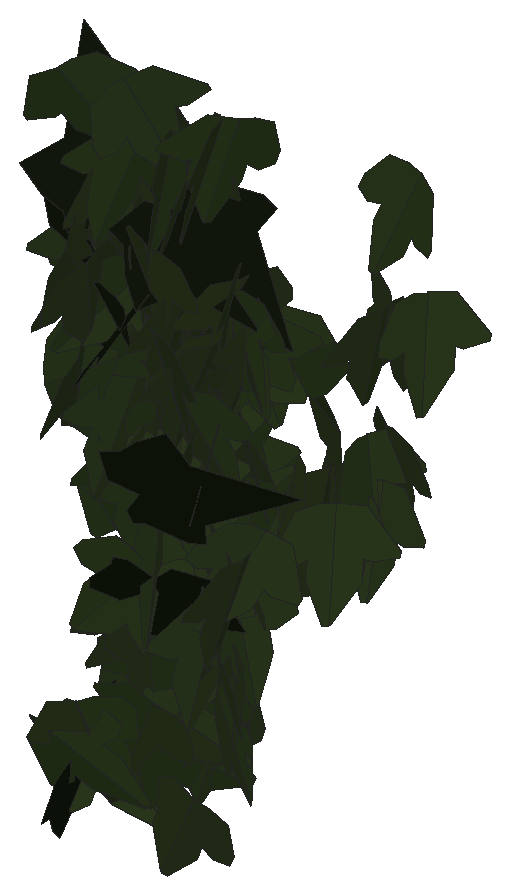
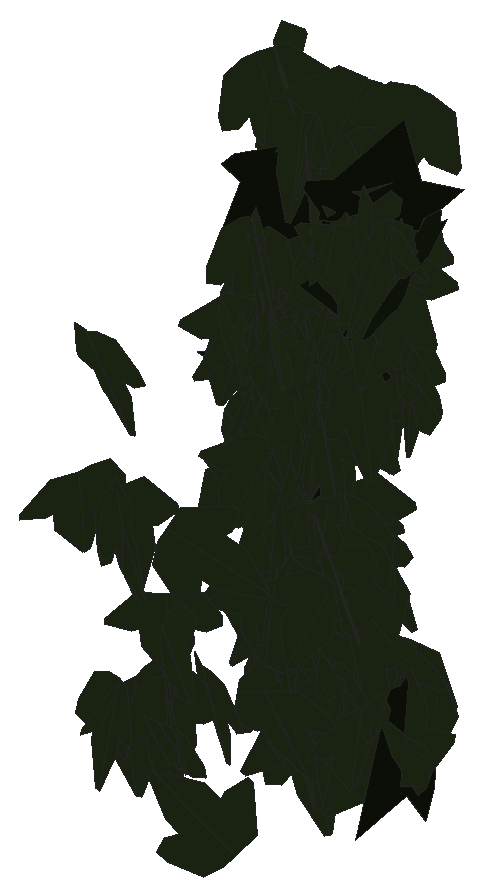
# SketchUp Ruby script. Lengths in inches.
U = 1.inch
M = Sketchup.active_model
def pt(a) = Geom::Point3d.new(a.map { |v| v * U })
def face(e, loops, mat)
  f = e.add_face(loops[0].map { |a| pt(a) })
  loops[1..].each { |l| e.add_face(l.map { |a| pt(a) }).erase! }
  f.material = f.back_material = mat if mat
  f
end
# faces: each face lists its corners as indices into pts; further lists are holes
def faces(e, pts, list, mat = nil) = list.each { |f| face(e, (f[0].is_a?(Array) ? f : [f]).map { |l| l.map { |i| pts[i] } }, mat) }
# xy, xz, yz: faces in a plane at the given z, y or x. An outline is a flat list of corners, or four numbers for a rectangle; further outlines are holes
def ring(l) = l.size == 4 ? [[l[0], l[1]], [l[2], l[1]], [l[2], l[3]], [l[0], l[3]]] : l.each_slice(2).to_a
def flat(e, list, mat, &to3) = list.each { |f| face(e, (f[0].is_a?(Array) ? f : [f]).map { |l| ring(l).map { |u, v| to3.(u, v) } }, mat) }
def xy(e, z, list, mat = nil) = flat(e, list, mat) { |x, y| [x, y, z] }
def xz(e, y, list, mat = nil) = flat(e, list, mat) { |x, z| [x, y, z] }
def yz(e, x, list, mat = nil) = flat(e, list, mat) { |y, z| [x, y, z] }
def lines(e, pts, list) = list.each { |a, b| e.add_line(pt(pts[a]), pt(pts[b])) }
# prism: a flat outline (further loops are holes) pulled along v
def prism(e, loops, v, mat = nil)
  f = face(e, loops, mat); d = Geom::Vector3d.new(v.map { |x| x * U })
  f.pushpull(f.normal.samedirection?(d) ? d.length : -d.length)
end
def box(e, o, s, mat = nil) = prism(e, [[o, [o[0] + s[0], o[1], o[2]], [o[0] + s[0], o[1] + s[1], o[2]], [o[0], o[1] + s[1], o[2]]]], [0, 0, s[2]], mat)
def at(x, y, z, deg = 0) = Geom::Transformation.translation(pt([x, y, z])) * Geom::Transformation.rotation(ORIGIN, Z_AXIS, deg.degrees)
def axes(o, x, y, z) = Geom::Transformation.new([*x, 0, *y, 0, *z, 0, *pt(o).to_a, 1])
def part(name) = M.definitions.add(name)
# library, detail: a bought-in or finely detailed component or shape, given as its bounding box
def library(name, o, s) = part(name).tap { |d| box(d.entities, o, s) }
def detail(e, o, s) = box(e.add_group.entities, o, s)
def put(e, d, t, mat = nil) = e.add_instance(d, t).tap { |i| i.material = mat if mat }
def group(e, t, mat = nil) = e.add_group.tap { |g| g.transformation = t; g.material = mat if mat }.entities
root = M.entities
M.materials.add("efeu1").color = [18, 25, 13]
M.materials.add("efeu2").color = [43, 57, 29]
c1 = part("ivyleaf_10")
p = [[0,0.5,-0.03],[-0.0625,2.02,-0.43],[-0.19,2.01,-0.46],[-0.54,1.05,-0.29],[-0.52,0.625,-0.18],[-0.83,0.76,-0.28],
  [-1.16,0.64,-0.33],[-1.15,0.33,-0.24],[-0.77,-0.39,0.02],[-0.3,-0.51,0.16],[0.04,-0.48,0.23],[-0.02,2.01,-0.4375],
  [-0.06,2.01,-0.43],[0.04,-0.49,0.23],[0.67,-0.49,0.14],[1.38,0.36,-0.2],[1.375,0.51,-0.24],[0.81,0.65,-0.19],
  [0.62,0.59,-0.15],[0.6,1.09,-0.28],[0.5,1.23,-0.31]]
faces(c1.entities,p,[[0,1,2,3,4,5,6,7,8,9,10],[11,12,0,13,14,15,16,17,18,19,20]],"efeu2")
c2 = part("ivyleaf_9")
p = [[1.54,2.16,1.25],[1.36,2.04,1.19],[-0.21,0.99,0.68],[-0.71,1.11,0.82],[-0.85,0.86,0.67],[-0.8,0.17,0.21],
  [-0.9,-0.01,0.1],[-0.67,-0.16,-0.02],[-0.08,-0.08,-0.05],[-0.03,-0.6,-0.4],[0.65,-0.88,-0.66],[0.83,-0.6,-0.49],
  [1.29,-0.42,-0.43],[1.8125,-0.07,-0.26],[1.21,0.44,0.15]]
faces(c2.entities,p,[[0,1,2,3,4,5,6,7,8,9,10,11,12,13,14]],"efeu1")
put(root,c1,axes([524.13,137.27,180.83],[-0.47127,-0.50798,0.10975],[-0.01474,-0.13503,-0.68828],[0.51949,-0.46466,0.08003]))
put(root,c1,axes([523.68,138.11,176.34],[-0.41982,-0.07668,-0.5031],[0.50786,-0.0214,-0.42054],[0.03256,-0.6549,0.07265]))
put(root,c2,axes([524.28,136.52,173],[-0.12797,0.15475,-0.77354],[-0.54598,0.54826,0.2],[0.5694,0.56049,0.01793]))
put(root,c1,axes([524.01,137.43,181.48],[0.01965,-0.59176,-0.37503],[0.17898,0.36697,-0.56966],[0.67734,-0.0798,0.16141]))
put(root,c1,axes([524.07,137.33,180.49],[-0.68472,-0.08826,-0.11103],[0.10971,0.01732,-0.69037],[0.08989,-0.69344,-0.00311]))
put(root,c1,axes([523.99,138.14,173.87],[0.1027,0.64813,-0.05276],[-0.00224,-0.05306,-0.65619],[-0.65027,0.10254,-0.00607]))
put(root,c1,axes([523.99,136.84,183.39],[-0.56307,-0.26725,-0.35085],[0.30678,0.17146,-0.62295],[0.31687,-0.6409,-0.02035]))
put(root,c1,axes([524.22,137.85,177.24],[-0.16103,-0.65598,0.03364],[0.00261,-0.03527,-0.67537],[0.65684,-0.16068,0.01093]))
put(root,c1,axes([523.81,141.61,173.5],[-0.25496,-0.47153,0.39714],[0.4117,0.18966,0.48949],[-0.45888,0.43215,0.2185]))
put(root,c2,axes([523.69,137.33,181.05],[0.37757,-0.64527,0.24174],[0.1234,-0.20787,-0.74761],[0.67792,0.39722,0.00145]))
put(root,c1,axes([523.91,138.54,175.84],[0.61685,-0.44004,-0.21224],[0.17432,-0.1211,0.75771],[-0.45639,-0.641,0.00255]))
put(root,c1,axes([524.28,137.875,174.81],[-0.23021,-0.6301,0.0833],[-0.03597,-0.07554,-0.67079],[0.63456,-0.23287,-0.0078]))
put(root,c1,axes([524.3,136.48,179.13],[0.1386,-0.62847,-0.31118],[-0.0449,0.3086,-0.64325],[0.69985,0.14426,0.02036]))
put(root,c1,axes([524.3,137.66,179.06],[-0.17806,-0.66496,0.00959],[0.0095,-0.01247,-0.68827],[0.66496,-0.17789,0.01241]))
put(root,c1,axes([524.14,136.92,172.63],[-0.65895,0.03998,0.2448],[0.22783,-0.17716,0.64222],[0.09807,0.68027,0.15286]))
put(root,c1,axes([523.75,138.12,176.41],[-0.06964,0.00974,-0.65545],[0.65142,-0.07253,-0.07029],[-0.07316,-0.65513,-0.00197]))
put(root,c1,axes([524.74,137.22,181.56],[0.27108,-0.01403,-0.65537],[-0.62637,0.20358,-0.26344],[0.1933,0.67937,0.06541]))
put(root,c1,axes([524.04,137.99,177.01],[-0.53798,0.00696,-0.38476],[0.38082,-0.08551,-0.53402],[-0.05536,-0.65586,0.06554]))
put(root,c2,axes([524.57,137.22,181.8],[-0.66535,-0.37347,0.21608],[0.2123,0.06237,0.76151],[-0.37563,0.69677,0.04765]))
put(root,c1,axes([523.84,136.8125,178.71],[0.35281,-0.17142,-0.59477],[0.52234,-0.28486,0.39195],[-0.3321,-0.63015,-0.01539]))
put(root,c1,axes([524.32,138.11,174.26],[-0.02917,0.66023,0.00732],[-0.00015,0.00732,-0.66088],[-0.66027,-0.02917,-0.00017]))
put(root,c1,axes([524.48,136.12,181.14],[0.05796,-0.52571,-0.47393],[0.0138,0.47626,-0.52661],[0.70766,0.03377,0.04909]))
put(root,c1,axes([524.47,137.02,182.01],[0.0661,-0.70793,-0.03914],[0.10727,0.04884,-0.70226],[0.70085,0.0593,0.11118]))
put(root,c1,axes([524.11,137.17,172.91],[0.40201,0.41206,0.50055],[0.36329,0.34465,-0.57549],[-0.537,0.54164,-0.01461]))
put(root,c1,axes([524.46,140.96,175.57],[0.5682,-0.33434,0.00262],[0.01542,0.02105,-0.65876],[0.334,0.56781,0.02596]))
put(root,c1,axes([524.86,141.36,176.31],[0.17116,-0.02559,-0.66433],[-0.41191,0.53438,-0.12671],[0.52184,0.4302,0.11788]))
put(root,c1,axes([524.68,137.73,176.86],[-0.5354,-0.36098,0.13926],[-0.07833,-0.13172,-0.64255],[0.3789,-0.5373,0.06395]))
put(root,c1,axes([524.94,140.9375,177.72],[-0.25032,-0.20862,0.59666],[-0.43778,-0.40569,-0.32551],[0.45594,-0.50407,0.01504]))
put(root,c1,axes([524.64,136.28,180.8],[-0.08644,-0.67752,-0.19305],[0.0169,0.19245,-0.68297],[0.70428,-0.08778,-0.00731]))
put(root,c1,axes([524.91,137.4,178.67],[0.44668,0.24064,-0.45675],[-0.51431,0.15486,-0.42138],[-0.04493,0.61981,0.28262]))
put(root,c1,axes([524.875,136.99,180.42],[0.32019,0.39936,-0.48285],[-0.4694,-0.20633,-0.48192],[-0.41509,0.54138,0.17251]))
put(root,c1,axes([524.67,137.52,174.83],[-0.2341,-0.60072,-0.16652],[0.07404,0.14982,-0.64457],[0.61896,-0.24513,0.01412]))
put(root,c1,axes([524.69,139.15,174.3],[0.62585,0.0799,-0.18006],[-0.17726,-0.03317,-0.63085],[-0.08593,0.65039,-0.01006]))
put(root,c1,axes([524.4,138.35,175.875],[0.48196,0.33142,0.29887],[0.18614,0.25052,-0.57796],[-0.40561,0.50877,0.0899]))
put(root,c1,axes([524.24,136.31,173.43],[-0.42737,0.04164,-0.59608],[0.59625,-0.0183,-0.42877],[-0.03915,-0.73323,-0.02315]))
put(root,c1,axes([524.625,136.36,173.83],[-0.63833,-0.27201,-0.18089],[0.16459,0.07519,-0.69386],[0.28218,-0.65919,-0.0045]))
put(root,c1,axes([524.28,138.12,174.2],[0.50108,-0.13334,-0.40925],[0.41514,-0.01619,0.51356],[-0.1137,-0.64677,0.07152]))
put(root,c1,axes([524.95,136.83,175.92],[0.54984,-0.14115,-0.43031],[-0.40676,0.14363,-0.56686],[0.19909,0.68327,0.03027]))
put(root,c1,axes([524.74,137.08,178.53],[-0.13928,-0.63759,0.28466],[0.06944,-0.30148,-0.64128],[0.69479,-0.09769,0.12115]))
put(root,c1,axes([524.83,137.78,178.33],[0.47446,-0.36241,-0.31904],[-0.17468,0.28816,-0.5871],[0.45012,0.49382,0.10845]))
put(root,c1,axes([524.85,137.07,182.5],[-0.26745,-0.59595,0.26997],[-0.02091,-0.28371,-0.64702],[0.65391,-0.25282,0.08972]))
put(root,c1,axes([524.87,141.47,175.38],[-0.26919,-0.62282,-0.03193],[0.01265,0.02931,-0.6785],[0.62351,-0.26949,-0.00002]))
put(root,c1,axes([524.69,141.53,175.25],[0.40619,-0.50539,0.20075],[0.19133,-0.10173,-0.64323],[0.50903,0.44152,0.08159]))
put(root,c1,axes([524.92,137.6,177.89],[-0.04006,-0.66463,-0.04561],[0.00981,0.0451,-0.6658],[0.66612,-0.04064,0.00706]))
put(root,c2,axes([524.93,136.34,179.73],[-0.36725,0.64319,-0.28504],[-0.14329,0.24642,0.74065],[0.68877,0.39421,0.0021]))
put(root,c1,axes([524.55,137.43,181.07],[0.32127,0.31857,0.53996],[0.344,0.41766,-0.45109],[-0.52412,0.4694,0.03491]))
put(root,c1,axes([524.77,138.07,176.62],[-0.57148,0.13894,-0.30268],[0.29477,-0.06878,-0.58812],[-0.15502,-0.64302,-0.00249]))
put(root,c1,axes([524.95,137.26,181.38],[-0.14844,0.67141,-0.15233],[-0.05007,-0.16594,-0.68263],[-0.68665,-0.13305,0.08271]))
put(root,c1,axes([525.1,137.49,174.53],[-0.57497,-0.34902,-0.06739],[0.05626,0.03718,-0.6726],[0.35098,-0.57771,-0.00258]))
put(root,c1,axes([524.93,141.625,174.82],[0.67325,-0.01571,0.05918],[0.05922,0.0013,-0.67343],[0.01554,0.67584,0.00267]))
put(root,c1,axes([525.18,142.4,175.68],[-0.60349,0.29947,0.08062],[-0.08495,0.01002,-0.6731],[-0.29827,-0.60877,0.02858]))
put(root,c1,axes([525.18,137.68,179.22],[-0.37765,-0.57098,0.05906],[0.02525,-0.08715,-0.6811],[0.57348,-0.37217,0.06888]))
put(root,c1,axes([525.41,136.76,173.95],[-0.58601,-0.11328,0.30476],[-0.30295,-0.0378,-0.59658],[0.11803,-0.65943,-0.01815]))
put(root,c1,axes([524.97,136.96,183.38],[0.43099,0.45239,0.33799],[0.04653,0.39528,-0.58841],[-0.56279,0.37913,0.21019]))
put(root,c1,axes([525.28,137.01,174.83],[-0.64634,-0.13021,0.09156],[-0.08979,-0.01792,-0.65933],[0.13143,-0.65255,-0.00016]))
put(root,c1,axes([525.1875,137.66,178.46],[-0.31192,-0.60076,-0.06235],[0.06327,0.03728,-0.6758],[0.60066,-0.3159,0.03881]))
put(root,c1,axes([525.24,137.2,179.1],[-0.28825,0.57807,0.22661],[-0.12516,0.19062,-0.64545],[-0.60816,-0.31322,0.02543]))
put(root,c1,axes([525.23,138.06,173.37],[0.37959,-0.54386,-0.02655],[-0.01761,0.02009,-0.66322],[0.54422,0.37999,-0.00294]))
put(root,c1,axes([525.34,137.98,175.42],[0.22222,0.59015,0.22223],[-0.07503,-0.20921,0.63059],[0.62612,-0.23452,-0.00331]))
put(root,c1,axes([525.1875,141.89,175.63],[0.06861,0.67305,-0.08399],[-0.00405,-0.08401,-0.67652],[-0.67826,0.06859,-0.00446]))
put(root,c1,axes([525.34,137.22,179.82],[-0.35603,0.5905,0.14518],[-0.10274,0.1074,-0.68879],[-0.59934,-0.36919,0.03183]))
put(root,c1,axes([525.37,137.5,179.64],[0.40288,-0.5514,-0.11074],[-0.01717,0.1241,-0.68038],[0.56215,0.39897,0.05859]))
put(root,c1,axes([525.61,138.21,176.51],[-0.62264,0.36924,0.3488],[-0.30682,0.16635,-0.7238],[-0.4048,-0.69403,0.01209]))
put(root,c1,axes([525.24,137.5,178.85],[0.68007,-0.01999,0.0766],[0.07912,0.14965,-0.66341],[0.00263,0.66781,0.15096]))
put(root,c1,axes([525.24,138.54,175.71],[0.49923,0.42513,0.07231],[0.0525,0.04988,-0.65571],[-0.42802,0.50197,0.00391]))
put(root,c2,axes([525.53,136.73,176.1],[0.51854,0.41964,-0.39361],[-0.31934,-0.23085,-0.66682],[-0.47859,0.60871,0.01846]))
put(root,c1,axes([525.3125,141.82,175],[0.67617,0.00904,0.05914],[0.0592,-0.0039,-0.67621],[-0.00866,0.67874,-0.00467]))
put(root,c1,axes([525.53,137.57,179.51],[0.09045,-0.68841,-0.00253],[-0.01556,0.00051,-0.69416],[0.68824,0.09049,-0.01536]))
put(root,c1,axes([525.47,137.86,177.83],[-0.61822,0.25026,-0.0324],[0.02921,-0.01419,-0.66695],[-0.25065,-0.61891,0.00219]))
put(root,c1,axes([525.65,136.49,181.29],[-0.66853,0.11193,0.15883],[-0.15813,0.01729,-0.67778],[-0.11291,-0.68692,0.00882]))
put(root,c1,axes([525.9,141.4375,178.15],[-0.38055,0.20234,0.54537],[-0.54217,0.11275,-0.42015],[-0.21076,-0.65539,0.09609]))
put(root,c1,axes([525.52,137.61,179.57],[-0.58588,-0.32862,-0.12945],[0.1454,0.00409,-0.66847],[0.32188,-0.6,0.06634]))
put(root,c1,axes([525.66,137.11,182.16],[0.22405,-0.5516,-0.38764],[-0.11992,0.36937,-0.59491],[0.66344,0.25305,0.02338]))
put(root,c1,axes([525.87,137.07,172.46],[-0.612,-0.05726,0.34253],[-0.33934,-0.04897,-0.61449],[0.07384,-0.69962,0.01498]))
put(root,c1,axes([525.78,138,175.77],[-0.60819,0.20798,0.18361],[-0.18675,0.02026,-0.64154],[-0.20517,-0.63498,0.03967]))
put(root,c1,axes([525.67,137.01,180.35],[0.05569,-0.70385,0.02087],[-0.00142,-0.02105,-0.70604],[0.70416,0.05562,-0.00307]))
put(root,c1,axes([525.52,137.21,177.55],[0.66391,0.24782,-0.06113],[0.05609,0.02453,0.70865],[0.24901,-0.66627,0.00335]))
put(root,c1,axes([525.37,136.84,176.63],[0.48175,-0.33325,0.38155],[0.31451,-0.21603,-0.58578],[0.39714,0.57532,0.00105]))
put(root,c1,axes([525.59,137.01,182.65],[-0.14898,0.5728,-0.39445],[-0.04156,-0.41001,-0.5797],[-0.69423,-0.09838,0.11935]))
put(root,c1,axes([525.78,137.33,182.8],[-0.66495,0.20978,0.13214],[-0.13316,0.01687,-0.69686],[-0.20914,-0.67774,0.02356]))
put(root,c1,axes([525.73,141.32,178.19],[-0.05396,-0.66383,0.00555],[0.01079,-0.00644,-0.66592],[0.66376,-0.05386,0.01127]))
put(root,c1,axes([525.7,137.68,179.54],[0.21013,-0.64611,0.10223],[0.01499,-0.10259,-0.6792],[0.65397,0.20995,-0.01727]))
put(root,c1,axes([525.51,137.23,173.26],[-0.26628,-0.36141,-0.54956],[0.33465,0.43598,-0.44886],[0.56626,-0.4276,0.00684]))
put(root,c1,axes([525.8,137.23,179.59],[-0.26778,0.46878,0.42568],[-0.2043,0.3735,-0.53984],[-0.59935,-0.33676,-0.00617]))
put(root,c1,axes([525.8,137.24,178.33],[0.30658,-0.61002,-0.07226],[-0.03993,0.0608,-0.68268],[0.61299,0.30905,-0.00833]))
put(root,c1,axes([525.88,137.67,173.65],[-0.33079,-0.59425,0.12127],[-0.04407,-0.11421,-0.67991],[0.6049,-0.33329,0.01678]))
put(root,c1,axes([525.55,137.48,175.71],[0.65485,0.18999,0.14129],[0.13669,0.03595,-0.68184],[-0.19333,0.66895,-0.00349]))
put(root,c1,axes([525.7,138,176.03],[0.41575,-0.50314,0.14382],[0.12256,-0.08495,-0.6515],[0.50874,0.43164,0.03942]))
put(root,c1,axes([525.35,137.18,173.89],[-0.26738,-0.01656,-0.65176],[0.64791,-0.08527,-0.26363],[-0.07267,-0.6993,0.04759]))
put(root,c1,axes([525.93,137.4375,179.58],[-0.17391,-0.6615,0.03756],[0.01499,-0.04275,-0.6835],[0.66239,-0.17271,0.02533]))
put(root,c1,axes([525.78,137.39,176.72],[-0.54298,0.35357,-0.15906],[0.12351,-0.10172,-0.64772],[-0.3675,-0.55658,0.01734]))
put(root,c1,axes([525.87,136.48,179.96],[-0.55375,0.40391,-0.02683],[0.02737,-0.008,-0.68534],[-0.40388,-0.55434,-0.00966]))
put(root,c1,axes([525.9,137.67,179.46],[-0.19111,0.64566,0.03839],[-0.02024,0.03405,-0.67328],[-0.64648,-0.19193,0.00973]))
put(root,c1,axes([526.09,137,179.59],[-0.01669,-0.70495,0.14492],[-0.01441,-0.1446,-0.70507],[0.71955,-0.01925,-0.01076]))
put(root,c1,axes([525.89,137.68,178.79],[0.29463,-0.61908,-0.05153],[0.01056,-0.05203,0.6855],[-0.62113,-0.29454,-0.01279]))
put(root,c1,axes([525.83,137.95,177.53],[0.35191,0.48528,0.30599],[0.14282,0.27356,-0.59811],[-0.55564,0.37767,0.04006]))
put(root,c1,axes([526.12,137.4375,175.03],[-0.04264,-0.34561,-0.58866],[0.04428,0.58716,-0.34794],[0.68118,-0.0598,-0.01423]))
put(root,c1,axes([526.05,137.31,178.38],[0.43562,-0.50722,0.1045],[0.06347,-0.08323,-0.66858],[0.51396,0.44018,-0.006]))
put(root,c1,axes([526.32,137.37,174.65],[0.43473,-0.32539,-0.48302],[-0.30526,0.38602,-0.53477],[0.49599,0.52277,0.09424]))
put(root,c1,axes([526.11,137.21,175.36],[-0.17833,-0.63529,0.24202],[0.12265,-0.27617,-0.63455],[0.66867,-0.11878,0.18094]))
put(root,c1,axes([526.19,137.8125,179.47],[0.11487,-0.66534,0.07138],[-0.00304,-0.07295,-0.67501],[0.66915,0.11389,-0.01532]))
put(root,c1,axes([526.3,137.59,179.57],[0.61849,-0.11408,-0.25369],[-0.23239,0.12799,-0.62411],[0.15287,0.65613,0.07764]))
put(root,c2,axes([525.8125,137,181.8125],[-0.09468,-0.33999,-0.74396],[0.29876,0.68281,-0.35007],[0.76145,-0.31018,0.04485]))
put(root,c1,axes([526.09,136.84,178.94],[-0.64865,0.03739,-0.22953],[0.22981,-0.00107,-0.64962],[-0.03561,-0.68806,-0.01146]))
put(root,c1,axes([526.59,137.62,177.68],[0.23101,-0.04064,-0.63355],[-0.51062,0.38871,-0.21112],[0.37723,0.55105,0.1022]))
put(root,c1,axes([526.13,139.87,175.77],[0.52398,0.41506,-0.01188],[-0.01038,-0.00603,-0.66845],[-0.4151,0.52408,0.00172]))
put(root,c1,axes([526.23,137.83,179.25],[0.37879,0.52939,-0.18848],[-0.12271,-0.14389,-0.65077],[-0.54838,0.39787,0.01543]))
put(root,c1,axes([526.37,141.17,180.56],[0.63058,-0.23106,-0.15832],[-0.15172,0.04606,-0.67153],[0.23544,0.64852,-0.00872]))
put(root,c1,axes([526.46,137.15,174.88],[-0.36807,0.50743,0.34833],[-0.22909,0.26376,-0.62629],[-0.57126,-0.43271,0.02672]))
put(root,c1,axes([526.3,137.5,180.82],[0.3752,-0.58849,0.03217],[0.05858,-0.00071,-0.69621],[0.58645,0.37658,0.04896]))
put(root,c1,axes([526.4375,137.33,180.51],[-0.68558,0.0927,0.02838],[-0.03586,-0.05418,-0.68934],[-0.09007,-0.68402,0.05844]))
put(root,c1,axes([526.53,137.15,183.27],[-0.38089,-0.58178,0.17553],[-0.07122,-0.163,-0.69478],[0.60349,-0.38642,0.02879]))
put(root,c1,axes([526.16,137.29,176.86],[0.1657,0.24204,-0.60453],[0.34197,0.49851,0.29333],[0.55417,-0.38,-0.00025]))
put(root,c1,axes([526.29,137.64,175.49],[0.0784,0.66805,0.02246],[0.00457,0.02208,-0.67263],[-0.66841,0.07851,-0.00197]))
put(root,c1,axes([526.49,137.4,180.67],[-0.33266,-0.61988,-0.05908],[0.0353,0.0481,-0.70345],[0.62169,-0.33442,0.00833]))
put(root,c2,axes([525.79,136.18,177.83],[0.35419,-0.04591,0.68883],[0.6869,-0.05393,-0.35679],[0.06899,0.77268,0.01602]))
put(root,c1,axes([526.34,137.74,178.41],[-0.30725,0.59234,-0.09201],[0.05652,-0.0743,-0.6671],[-0.59678,-0.312,-0.01581]))
put(root,c1,axes([526.3,137.8125,179.61],[0.40556,0.49376,0.23251],[0.01525,0.27931,-0.61975],[-0.54555,0.37487,0.15552]))
put(root,c1,axes([526.51,137.76,179.84],[0.09677,-0.62053,0.2652],[0.03104,-0.26354,-0.62796],[0.67411,0.10121,-0.00915]))
put(root,c1,axes([526.4375,141.55,178.45],[0.30069,0.59214,-0.09712],[-0.02908,-0.09412,-0.6639],[-0.59935,0.30164,-0.01651]))
put(root,c1,axes([526.49,136.68,183.35],[0.3765,-0.59287,0.16432],[0.07375,-0.14776,-0.70212],[0.61078,0.3833,-0.01651]))
put(root,c1,axes([526.6,137.07,176.36],[0.07592,-0.70488,0.09799],[0.02029,-0.09636,-0.70889],[0.71137,0.07798,0.00976]))
put(root,c1,axes([526.35,137.55,180.3],[-0.49085,0.27056,-0.40221],[0.26797,-0.32555,-0.54601],[-0.40394,-0.54473,0.12654]))
put(root,c1,axes([526.72,137.35,176.72],[0.45045,0.37582,-0.33486],[-0.31477,-0.14034,-0.58094],[-0.39279,0.54345,0.08154]))
put(root,c1,axes([526.57,137.01,174.27],[-0.25815,0.63815,0.07496],[-0.02916,0.06906,-0.68838],[-0.64187,-0.25979,0.00113]))
